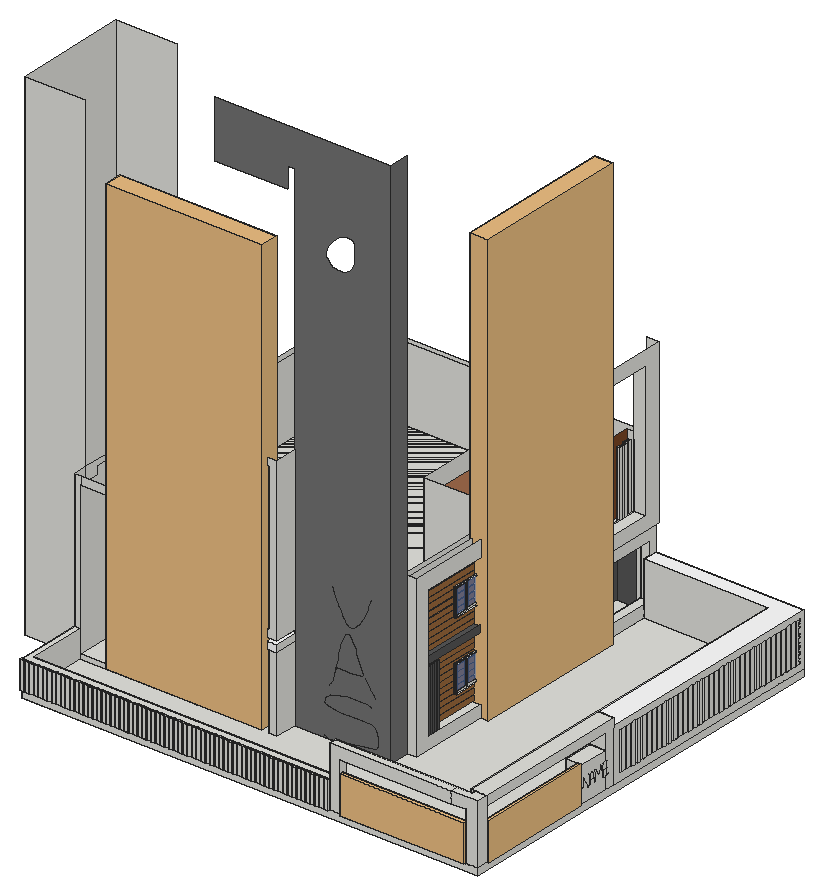
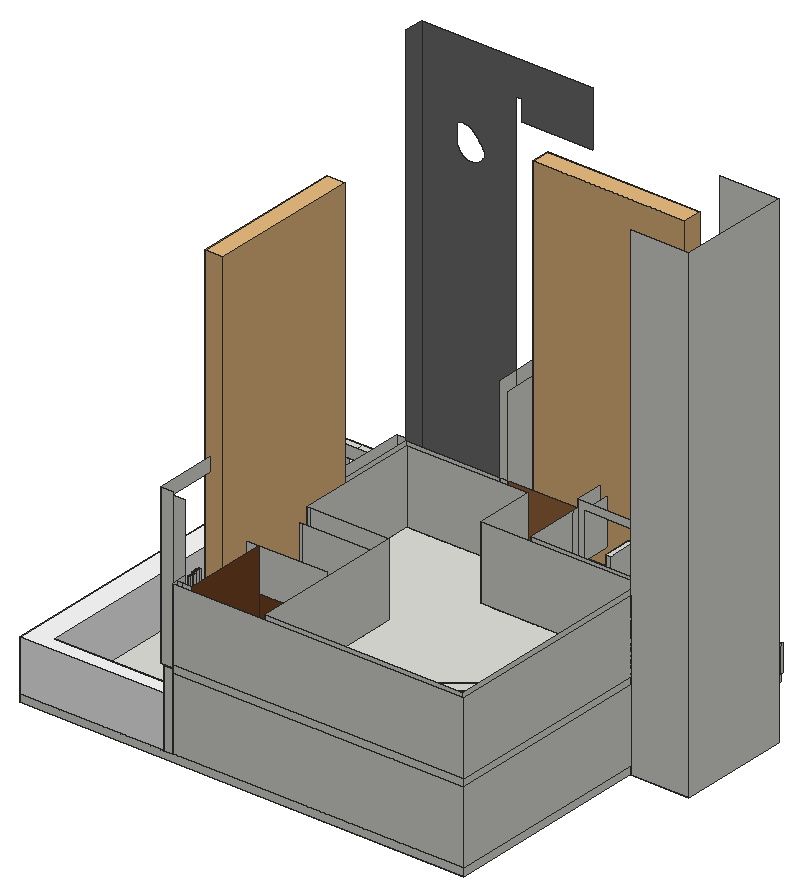
# SketchUp Ruby script. Lengths in inches.
U = 1.inch
M = Sketchup.active_model
def pt(a) = Geom::Point3d.new(a.map { |v| v * U })
def face(e, loops, mat)
  f = e.add_face(loops[0].map { |a| pt(a) })
  loops[1..].each { |l| e.add_face(l.map { |a| pt(a) }).erase! }
  f.material = f.back_material = mat if mat
  f
end
# faces: each face lists its corners as indices into pts; further lists are holes
def faces(e, pts, list, mat = nil) = list.each { |f| face(e, (f[0].is_a?(Array) ? f : [f]).map { |l| l.map { |i| pts[i] } }, mat) }
# xy, xz, yz: faces in a plane at the given z, y or x. An outline is a flat list of corners, or four numbers for a rectangle; further outlines are holes
def ring(l) = l.size == 4 ? [[l[0], l[1]], [l[2], l[1]], [l[2], l[3]], [l[0], l[3]]] : l.each_slice(2).to_a
def flat(e, list, mat, &to3) = list.each { |f| face(e, (f[0].is_a?(Array) ? f : [f]).map { |l| ring(l).map { |u, v| to3.(u, v) } }, mat) }
def xy(e, z, list, mat = nil) = flat(e, list, mat) { |x, y| [x, y, z] }
def xz(e, y, list, mat = nil) = flat(e, list, mat) { |x, z| [x, y, z] }
def yz(e, x, list, mat = nil) = flat(e, list, mat) { |y, z| [x, y, z] }
def lines(e, pts, list) = list.each { |a, b| e.add_line(pt(pts[a]), pt(pts[b])) }
# prism: a flat outline (further loops are holes) pulled along v
def prism(e, loops, v, mat = nil)
  f = face(e, loops, mat); d = Geom::Vector3d.new(v.map { |x| x * U })
  f.pushpull(f.normal.samedirection?(d) ? d.length : -d.length)
end
def box(e, o, s, mat = nil) = prism(e, [[o, [o[0] + s[0], o[1], o[2]], [o[0] + s[0], o[1] + s[1], o[2]], [o[0], o[1] + s[1], o[2]]]], [0, 0, s[2]], mat)
def at(x, y, z, deg = 0) = Geom::Transformation.translation(pt([x, y, z])) * Geom::Transformation.rotation(ORIGIN, Z_AXIS, deg.degrees)
def axes(o, x, y, z) = Geom::Transformation.new([*x, 0, *y, 0, *z, 0, *pt(o).to_a, 1])
def part(name) = M.definitions.add(name)
# library, detail: a bought-in or finely detailed component or shape, given as its bounding box
def library(name, o, s) = part(name).tap { |d| box(d.entities, o, s) }
def detail(e, o, s) = box(e.add_group.entities, o, s)
def put(e, d, t, mat = nil) = e.add_instance(d, t).tap { |i| i.material = mat if mat }
def group(e, t, mat = nil) = e.add_group.tap { |g| g.transformation = t; g.material = mat if mat }.entities
root = M.entities
M.materials.add("[Color M00]").color = [255, 255, 255]
M.materials.add("[Color M05]").color = [114, 114, 114]
M.materials.add("[Color M06]").color = [86, 86, 86]
M.materials.add("[Translucent Glass Blue]").color = [100, 149, 237]
M.materials["[Translucent Glass Blue]"].alpha = 0.5
M.materials.add("[Translucent_Glass_Gray]").color = [128, 128, 128]
M.materials["[Translucent_Glass_Gray]"].alpha = 0.5
M.materials.add("[Wood Floor]").color = [155, 105, 61]
M.materials.add("[Wood Veneer 01]").color = [120, 70, 37]
M.materials.add("[Wood Veneer 02]").color = [190, 128, 91]
c1 = library("House+plant_11",[-42.36,19.93,-20.98],[140.22,29.68,697.18])
c2 = part("Group\#13")
box(c2.entities,[0,-2.9375,0],[6.66,2.9375,44.375])
c3 = library("Group\#1076",[0,-1.74,0],[119.75,5.32,60.06])
c4 = part("Slatted corner screen")
put(c4.entities,c3,axes([-115.39,-96.71,0],[0,1.55247,0],[-1,0,0],[0,0,1]))
put(c4.entities,c3,axes([-334.41,-117.1,0],[1.66331,0,0],[0,1,0],[0,0,1]))
c5 = part("Group\#5")
xy(c5.entities,0,[[0,0,3.25,201.7]])
xy(c5.entities,8.11,[[0,0,3.25,201.7]])
xz(c5.entities,201.7,[[0,0,3.25,8.11]])
yz(c5.entities,3.25,[[0,0,201.7,8.11]])
c6 = part("Janela aluminio")
xy(c6.entities,0,[[0,0,47.24,1.57],[23.62,1.57,47.24,2.76],[0,2.76,25.98,3.9375],[0,3.9375,47.24,5.91]])
xy(c6.entities,43.31,[[0,0,47.24,1.57],[23.62,1.57,47.24,2.76],[0,2.76,0,5.91,47.24,5.91,47.24,3.9375,25.98,3.9375,25.98,2.76],[25.98,2.76,47.24,3.9375]])
xz(c6.entities,1.57,[[0,0,23.62,0,23.62,41.34,21.26,41.34,21.26,1.97,1.97,1.97,1.97,41.34,23.62,41.34,23.62,43.31,0,43.31],[[23.62,0,47.24,43.31],[25.7,1.97,45.28,41.34]]])
xz(c6.entities,2.76,[[[0,0,23.62,43.31],[2.36,2.36,21.26,40.94]],[23.62,0,25.98,43.31]])
xz(c6.entities,2.76,[[2.36,2.36,21.26,40.94]],"[Translucent Glass Blue]")
xz(c6.entities,3.9375,[[25.98,0,25.98,2.36,44.88,2.36,44.88,40.94,25.98,40.94,25.98,43.31,47.24,43.31,47.24,0]])
xz(c6.entities,3.9375,[[25.98,2.36,44.88,40.94]],"[Translucent Glass Blue]")
yz(c6.entities,0,[[0,0,1.57,43.31],[2.76,0,5.91,43.31]])
yz(c6.entities,23.62,[[1.57,0,2.76,43.31]])
yz(c6.entities,25.98,[[2.76,0,3.9375,43.31]])
yz(c6.entities,47.24,[[0,0,1.57,43.31],[1.57,0,2.76,43.31],[3.9375,0,5.91,43.31]])
c7 = part("Window frame")
prism(c7.entities,[[[0,70.87,0],[0,0,0],[0,0,47.24],[0,70.87,47.24]],[[0,1.97,1.97],[0,68.9,1.97],[0,68.9,45.28],[0,1.97,45.28]]],[7.875,0,0])
c8 = part("Window sash")
xy(c8.entities,0,[[0,0,3.9375,16.73]])
xy(c8.entities,0.98,[[0,0.98,1.77,15.75],[1.77,0.98,2.85,15.75],[2.85,0.98,3.9375,15.75]])
xy(c8.entities,42.32,[[0,0.98,1.77,15.75],[1.77,0.98,2.85,15.75],[2.85,0.98,3.9375,15.75]])
xy(c8.entities,43.31,[[0,0,3.9375,16.73]])
xz(c8.entities,0,[[0,0,3.9375,43.31]])
xz(c8.entities,0.98,[[0,0.98,1.77,42.32],[1.77,0.98,2.85,42.32],[2.85,0.98,3.9375,42.32]])
xz(c8.entities,15.75,[[0,0.98,1.77,42.32],[1.77,0.98,2.85,42.32],[2.85,0.98,3.9375,42.32]])
xz(c8.entities,16.73,[[0,0,3.9375,43.31]])
yz(c8.entities,0,[[[0,0,16.73,43.31],[0.98,0.98,15.75,42.32]]])
yz(c8.entities,1.77,[[0.98,0.98,15.75,42.32]],"[Translucent_Glass_Gray]")
yz(c8.entities,2.85,[[0.98,0.98,15.75,42.32]],"[Translucent_Glass_Gray]")
yz(c8.entities,3.9375,[[[0,0,16.73,43.31],[0.98,0.98,15.75,42.32]]])
c9 = part("simple window")
p = [[0,68.9,1.97],[0,35.43,1.97]]
lines(c9.entities,p,[[0,1]])
put(c9.entities,c7,at(0,0,0))
put(c9.entities,c8,axes([1.14,52.17,1.97],[0.71,0,0],[0,1,0],[0,0,1]))
put(c9.entities,c8,axes([1.14,1.97,1.97],[0.71,0,0],[0,1,0],[0,0,1]))
put(c9.entities,c8,axes([3.9375,18.7,1.97],[0.71,0,0],[0,1,0],[0,0,1]))
put(c9.entities,c8,axes([3.9375,35.43,1.97],[0.71,0,0],[0,1,0],[0,0,1]))
c10 = part("Group\#4")
box(c10.entities,[0,-480,0],[480,480,12])
c11 = part("Group\#12")
box(c11.entities,[0,0,-113.625],[4.125,3.0625,113.625])
xy(root,-12,[[0,129.5,96.8125,313.4]])
xy(root,-12,[[421.4,144.25,576.8125,176.625]],"[Color M05]")
xy(root,0,[[96.8125,2.9375,96.8125,108.5,105.7,108.5,105.7,15,590.66,15,590.66,2.9375],[590.66,2.9375,607.16,15.25],[810,2.9375,829.0625,21.875],[96.8125,108.5,286.44,176.625],[[409.15,108.5,421.4,108.5,421.4,176.625,591.75,176.625,591.75,656.625,576.8125,656.625,576.8125,400.39,441.125,400.39,441.125,509.52,537.25,509.52,537.25,647.625,576.8125,647.625,576.8125,656.625,96.8125,656.625,96.8125,185.625,105.8125,185.625,105.8125,273.5625,293.58,273.5625,293.58,176.625,409.15,176.625],[368.4,185.625,368.4,282.5625,105.8125,282.5625,105.8125,647.625,432.125,647.625,432.125,391.39,567.8125,391.39,567.8125,185.625]],
  [96.8125,176.625,105.8125,185.625],[368.4,185.625,567.8125,185.625,567.8125,391.39,432.125,391.39,432.125,647.625,105.8125,647.625,105.8125,282.5625,368.4,282.5625],[802.8125,212.39,829.0625,260.08],[802.8125,260.08,829.0625,276.46],[441.125,400.39,567.8125,400.39,567.8125,647.625,537.25,647.625,537.25,509.52,551.125,509.52,551.125,496.2,441.125,496.2],
  [567.8125,400.39,576.8125,647.625],[591.75,632.64,790.44,656.625]])
xy(root,0,[[286.44,108.5,293.58,141.5625]],"[Color M00]")
xy(root,7.8125,[[107.25,108.5,293.58,108.5,293.58,185.625,96.8125,185.625,96.8125,176.75,107.25,176.75]])
xy(root,10.33,[[819.0625,286.78,819.0625,646.3,829.0625,646.3,829.0625,297.7,821.875,297.7,821.875,292.02,829.0625,292.02,829.0625,286.78],[821.875,292.02,829.0625,297.7]])
xy(root,18.83,[[576.8125,198.69,591.75,644.4375]])
xy(root,43,[[286.44,108.5,293.58,176.625]],"[Color M00]")
xy(root,44.375,[[96.8125,2.9375,590.66,2.9375,590.66,15,105.7,15,105.7,108.5,96.8125,108.5]])
xy(root,53.625,[[441.125,496.2,551.125,509.52]])
xy(root,56,[[802.8125,212.39,829.0625,260.08]])
xy(root,60.625,[[576.8125,386.37,591.75,400.39]])
xy(root,62.1875,[[238.96,108.5,248.39,176.625]],"[Color M00]")
xy(root,74.24,[[819.0625,286.78,829.0625,286.78,829.0625,292.02,821.875,292.02,821.875,297.7,829.0625,297.7,829.0625,646.3,819.0625,646.3],[821.875,292.02,829.0625,297.7]])
xy(root,77.84,[[607.16,2.9375,810,15.25]])
xy(root,81.34,[[802.8125,21.875,829.0625,260.08]])
xy(root,84.5625,[[790.44,276.46,790.44,632.64,591.75,632.64,591.75,656.625,829.0625,656.625,829.0625,276.46]],"[Color M00]")
xy(root,96.09,[[590.66,2.9375,786.3125,15.25],[786.3125,2.9375,829.0625,2.9375,829.0625,21.875,810,21.875,810,15.25,786.3125,15.25],[802.8125,21.875,829.0625,276.46]])
xy(root,105.25,[[576.8125,400.39,591.75,644.4375]])
xy(root,120,[[[409.15,108.5,421.4,108.5,421.4,176.625,576.8125,176.625,576.8125,400.39,441.125,400.39,441.125,509.52,537.25,509.52,537.25,647.625,576.8125,647.625,576.8125,656.625,96.8125,656.625,96.8125,176.75,105.8125,176.75,105.8125,273.5625,293.58,273.5625,293.58,176.625,409.15,176.625],[368.4,185.625,368.4,282.5625,105.8125,282.5625,105.8125,647.625,432.125,647.625,432.125,391.39,567.8125,391.39,567.8125,185.625]],[96.8125,176.625,105.8125,176.75]])
xy(root,120,[[248.39,108.5,409.15,176.625]],"[Color M00]")
xy(root,120,[[576.8125,198.69,589.375,386.37]],"[Color M06]")
xy(root,125.71,[[576.8125,386.37,591.75,656.625]])
xy(root,127.5625,[[576.8125,386.37,596.375,656.625]])
xy(root,132,[[[96.8125,176.625,105.8125,176.625,105.8125,273.5625,293.58,273.5625,293.58,176.625,576.8125,176.625,576.8125,400.39,441.125,400.39,441.125,509.52,552.625,509.52,552.625,647.625,576.8125,647.625,576.8125,656.625,96.8125,656.625],[368.4,185.625,368.4,282.5625,105.8125,282.5625,105.8125,647.625,432.125,647.625,432.125,391.39,567.8125,391.39,567.8125,185.625]],[105.8125,176.625,293.58,273.5625],[368.4,185.625,567.8125,185.625,567.8125,391.39,432.125,391.39,432.125,647.625,105.8125,647.625,105.8125,282.5625,368.4,282.5625],[441.125,400.39,567.8125,400.39,567.8125,647.625,552.625,647.625,552.625,509.52,441.125,509.52],[567.8125,400.39,576.8125,647.625]])
xy(root,132,[[238.96,108.5,421.4,176.625]],"[Color M00]")
xy(root,132,[[576.8125,198.69,589.375,386.37]],"[Color M06]")
xy(root,136.75,[[238.96,108.5,421.4,176.625]])
xy(root,148.6875,[[576.8125,400.39,596.375,631.75]])
xy(root,149.72,[[247.29,108.5,408.47,176.625]])
xy(root,175.98,[[294.92,105.68,282.85,105.86,283.87,173.99,295.94,173.81]])
xy(root,181.38,[[441.125,495.37,591.75,509.52]])
xy(root,192.45,[[576.8125,386.37,596.375,400.39]])
xy(root,200.03,[[238.96,108.5,247.29,176.625]])
xz(root,2.9375,[[96.8125,0,584,44.375],[590.66,0,607.16,0,607.16,77.84,786.3125,77.84,786.3125,96.09,590.66,96.09],[810,0,829.0625,0,829.0625,96.09,786.3125,96.09,786.3125,77.84,810,77.84]])
xz(root,15,[[105.7,0,590.66,44.375]])
xz(root,15.25,[[590.66,0,590.66,96.09,810,96.09,810,77.84,607.16,77.84,607.16,0]])
xz(root,21.875,[[810,0,829.0625,81.34],[802.8125,81.34,810,96.09],[810,81.34,829.0625,96.09]])
xz(root,108.5,[[105.7,0,286.44,0,286.44,7.8125,107.25,7.8125,107.25,264,96.8125,264,96.8125,44.375,105.7,44.375],[409.15,0,421.4,120],[238.96,136.75,421.4,136.75,421.4,396,238.96,396,238.96,328.5625,250.4375,328.5625,250.4375,384,408.47,384,408.47,149.72,247.29,149.72,247.29,200.03,238.96,200.03]])
xz(root,108.5,[[286.44,0,293.58,7.8125],[286.44,7.8125,293.58,43],[238.96,62.1875,238.96,132,421.4,132,421.4,120,248.39,120,248.39,62.1875]],"[Color M00]")
xz(root,129.5,[[0,-12,96.8125,792]])
xz(root,144.25,[[[421.4,-12,576.8125,-12,576.8125,859.0625,293.58,859.0625,293.58,767.74,411.47,767.74,411.47,801.24,421.4,801.24],[499.28,678.61,496.52,678.68,493.5,678.8,491.18,678.99,488.85,679.28,486.04,679.74,483.9,680.62,481.86,681.66,480.42,683.44,478.12,684.95,476.52,686.92,475.09,689.5,473.78,691.2,472.16,693.875,472.29,696.5,472.54,698.74,472.87,700.99,473.375,703.48,474.84,705.29,475.72,707.47,477,709.55,478.57,711.1,479.9,713.53,481.51,715.31,482.91,717.36,484.83,719.08,486.18,720.94,488.32,722.59,489.21,724.33,494.25,727.71,498.73,730.52,506.22,732.9,508.87,732.625,511.41,732.18,513.8,731.55,515.96,730.33,517.58,728.38,518.67,726.53,519.03,723.43,519.05,720.89,519.07,717.8,519.08,715.27,519.08,712.16,519.06,709.68,519.01,706.6,518.93,703.9,518.75,701.49,518.48,698.83,518.06,696.2,517.19,693.71,515.95,691.83,514.6,689.38,512.91,687.64,511.65,685.61,509.4,683.71,507.3125,682.48,504.6,680.79,502.39,679.59],[488.29,106.62,488.6,110.46,490.04,114.3,490.41,118.74,490.65,123.21,490.87,127.17,492.64,132.22,494.14,136.88,494.63,140.95,496.73,145.54,497.9,149.01,500.61,154.49,502.59,158.07,505.04,161.36,508.8,162.92,512.82,158.32,515.375,155.08,517.24,151.33,519.4,146.99,520.85,142.62,522.12,138.13,523.31,134.68,525.51,130.3,526.77,126.94,527.37,123.24,530.09,118.92,531.4,115.1,532.57,110.72,535.46,107.9,512.74,106.76,501.53,106.76],[551.45,10.1875,552.47,11.31,557.07,12]],[551.45,10.1875,557.07,12,552.47,11.31],[488.29,106.62,501.53,106.76,512.74,106.76,535.46,107.9,532.57,110.72,531.4,115.1,530.09,118.92,527.37,123.24,526.77,126.94,525.51,130.3,523.31,134.68,522.12,138.13,520.85,142.62,519.4,146.99,517.24,151.33,515.375,155.08,512.82,158.32,508.8,162.92,505.04,161.36,502.59,158.07,500.61,154.49,497.9,149.01,496.73,145.54,494.63,140.95,494.14,136.88,492.64,132.22,490.87,127.17,490.65,123.21,490.41,118.74,490.04,114.3,488.6,110.46]],"[Color M05]")
xz(root,176.625,[[421.4,-12,576.8125,0],[96.8125,0,105.8125,120],[421.4,0,576.8125,120],[576.8125,0,591.75,256.375],[96.8125,120,105.8125,132],
  [421.4,120,576.8125,132],[96.8125,132,105.8125,252],[421.4,132,576.8125,252],[238.96,136.75,238.96,200.03,247.29,200.03,247.29,149.72,293.58,149.72,293.58,136.75],[293.58,136.75,421.4,136.75,421.4,252,408.47,252,408.47,149.72,293.58,149.72]])
xz(root,176.625,[[238.96,62.1875,248.39,120]],"[Color M00]")
xz(root,176.625,[[293.58,0,409.15,120],[293.58,132,421.4,136.75],[293.58,149.72,408.47,252]],"[Wood Floor]")
xz(root,176.75,[[96.8125,7.8125,96.8125,120,105.8125,120,105.8125,264,107.25,264,107.25,7.8125]])
xz(root,185.625,[[96.8125,0,105.8125,7.8125],[105.8125,0,293.58,7.8125],[368.4,0,567.8125,120],[368.4,132,567.8125,252]])
xz(root,198.69,[[576.8125,18.83,576.8125,120,589.375,120,589.375,132,576.8125,132,576.8125,218.23,580.0625,218.23,580.0625,226.34,576.8125,226.34,576.8125,230.57,591.75,230.57,591.75,18.83],[576.8125,120,589.375,132],[576.8125,218.23,580.0625,226.34]])
xz(root,212.39,[[802.8125,0,829.0625,56]])
xz(root,260.08,[[802.8125,0,829.0625,56],[802.8125,56,829.0625,81.34]])
xz(root,273.5625,[[105.8125,0,293.58,120],[105.8125,132,293.58,252]])
xz(root,276.46,[[790.44,0,802.8125,84.5625],[802.8125,0,829.0625,84.5625],[802.8125,84.5625,829.0625,96.09]])
xz(root,282.5625,[[105.8125,0,368.4,120],[105.8125,132,368.4,252]])
xz(root,286.78,[[819.0625,10.33,829.0625,74.24]])
xz(root,292.02,[[821.875,10.33,829.0625,74.24]])
xz(root,297.7,[[821.875,10.33,829.0625,74.24]])
xz(root,302.39,[[821.875,10.33,829.0625,74.24]])
xz(root,308.08,[[821.875,10.33,829.0625,74.24]])
xz(root,312.77,[[821.875,10.33,829.0625,74.24]])
xz(root,313.4,[[0,-12,96.8125,792]])
xz(root,318.45,[[821.875,10.33,829.0625,74.24]])
xz(root,323.14,[[821.875,10.33,829.0625,74.24]])
xz(root,328.83,[[821.875,10.33,829.0625,74.24]])
xz(root,333.52,[[821.875,10.33,829.0625,74.24]])
xz(root,339.2,[[821.875,10.33,829.0625,74.24]])
xz(root,343.89,[[821.875,10.33,829.0625,74.24]])
xz(root,349.58,[[821.875,10.33,829.0625,74.24]])
xz(root,354.27,[[821.875,10.33,829.0625,74.24]])
xz(root,359.95,[[821.875,10.33,829.0625,74.24]])
xz(root,364.64,[[821.875,10.33,829.0625,74.24]])
xz(root,370.33,[[821.875,10.33,829.0625,74.24]])
xz(root,375.02,[[821.875,10.33,829.0625,74.24]])
xz(root,380.7,[[821.875,10.33,829.0625,74.24]])
xz(root,385.39,[[821.875,10.33,829.0625,74.24]])
xz(root,386.37,[[576.8125,60.625,591.75,60.625,591.75,125.71,589.375,125.71,589.375,120,576.8125,120],[576.8125,120,589.375,125.71],[576.8125,125.71,589.375,127.5625],[576.8125,127.5625,589.375,132],[589.375,127.5625,596.375,127.5625,596.375,192.45,576.8125,192.45,576.8125,132,589.375,132]])
xz(root,391.08,[[821.875,10.33,829.0625,74.24]])
xz(root,391.39,[[432.125,0,562.8125,120],[562.8125,0,567.8125,120],[432.125,132,562.8125,252],[562.8125,132,567.8125,252]])
xz(root,395.77,[[821.875,10.33,829.0625,74.24]])
xz(root,400.39,[[441.125,0,567.8125,120],[567.8125,0,576.8125,120],[576.8125,60.625,591.75,105.25],[441.125,132,567.8125,230.57],[567.8125,132,576.8125,230.57],
  [576.8125,148.6875,596.375,192.45]])
xz(root,401.45,[[821.875,10.33,829.0625,74.24]])
xz(root,406.14,[[821.875,10.33,829.0625,74.24]])
xz(root,411.83,[[821.875,10.33,829.0625,74.24]])
xz(root,416.52,[[821.875,10.33,829.0625,74.24]])
xz(root,422.2,[[821.875,10.33,829.0625,74.24]])
xz(root,426.89,[[821.875,10.33,829.0625,74.24]])
xz(root,432.58,[[821.875,10.33,829.0625,74.24]])
xz(root,437.27,[[821.875,10.33,829.0625,74.24]])
xz(root,442.95,[[821.875,10.33,829.0625,74.24]])
xz(root,447.64,[[821.875,10.33,829.0625,74.24]])
xz(root,453.33,[[821.875,10.33,829.0625,74.24]])
xz(root,458.02,[[821.875,10.33,829.0625,74.24]])
xz(root,463.7,[[821.875,10.33,829.0625,74.24]])
xz(root,468.39,[[821.875,10.33,829.0625,74.24]])
xz(root,474.08,[[821.875,10.33,829.0625,74.24]])
xz(root,478.77,[[821.875,10.33,829.0625,74.24]])
xz(root,484.45,[[821.875,10.33,829.0625,74.24]])
xz(root,489.14,[[821.875,10.33,829.0625,74.24]])
xz(root,494.83,[[821.875,10.33,829.0625,74.24]])
xz(root,495.37,[[441.125,181.38,591.75,230.57]])
xz(root,496.2,[[441.125,0,551.125,53.625]])
xz(root,499.52,[[821.875,10.33,829.0625,74.24]])
xz(root,505.2,[[821.875,10.33,829.0625,74.24]])
xz(root,509.52,[[441.125,0,537.25,53.625],[537.25,0,551.125,53.625],[441.125,181.38,552.625,252],[552.625,181.38,552.625,252,576.8125,252,576.8125,256.375,591.75,256.375,591.75,181.38]])
xz(root,509.52,[[441.125,53.625,537.25,120]],"[Color M06]")
xz(root,509.52,[[441.125,132,552.625,181.38]],"[Wood Veneer 01]")
xz(root,509.95,[[821.875,10.33,829.0625,74.24]])
xz(root,515.64,[[821.875,10.33,829.0625,74.24]])
xz(root,520.39,[[821.875,10.33,829.0625,74.24]])
xz(root,526.08,[[821.875,10.33,829.0625,74.24]])
xz(root,530.83,[[821.875,10.33,829.0625,74.24]])
xz(root,536.52,[[821.875,10.33,829.0625,74.24]])
xz(root,541.27,[[821.875,10.33,829.0625,74.24]])
xz(root,546.95,[[821.875,10.33,829.0625,74.24]])
xz(root,551.7,[[821.875,10.33,829.0625,74.24]])
xz(root,557.39,[[821.875,10.33,829.0625,74.24]])
xz(root,562.14,[[821.875,10.33,829.0625,74.24]])
xz(root,567.83,[[821.875,10.33,829.0625,74.24]])
xz(root,572.58,[[821.875,10.33,829.0625,74.24]])
xz(root,578.27,[[821.875,10.33,829.0625,74.24]])
xz(root,583.02,[[821.875,10.33,829.0625,74.24]])
xz(root,588.7,[[821.875,10.33,829.0625,74.24]])
xz(root,593.45,[[821.875,10.33,829.0625,74.24]])
xz(root,599.14,[[821.875,10.33,829.0625,74.24]])
xz(root,603.89,[[821.875,10.33,829.0625,74.24]])
xz(root,609.58,[[821.875,10.33,829.0625,74.24]])
xz(root,613.7,[[821.875,10.33,829.0625,74.24]])
xz(root,619.39,[[821.875,10.33,829.0625,74.24]])
xz(root,623.52,[[821.875,10.33,829.0625,74.24]])
xz(root,629.2,[[821.875,10.33,829.0625,74.24]])
xz(root,631.75,[[576.8125,148.6875,596.375,365.16]])
xz(root,632.64,[[591.75,0,790.44,84.5625]])
xz(root,633.33,[[821.875,10.33,829.0625,74.24]])
xz(root,639.02,[[821.875,10.33,829.0625,74.24]])
xz(root,643.14,[[821.875,10.33,829.0625,74.24]])
xz(root,644.4375,[[576.8125,18.83,591.75,105.25]])
xz(root,646.3,[[819.0625,10.33,829.0625,74.24]])
xz(root,647.625,[[105.8125,0,432.125,120],[567.8125,0,576.8125,120],[105.8125,132,432.125,252],[552.625,132,567.8125,252],[567.8125,132,576.8125,252]])
xz(root,647.625,[[537.25,0,567.8125,120]],"[Color M06]")
xz(root,648.83,[[821.875,10.33,829.0625,74.24]])
xz(root,656.625,[[96.8125,0,576.8125,120],[576.8125,0,591.75,125.71],[576.8125,127.5625,596.375,387.92],[96.8125,132,576.8125,252]])
xz(root,656.625,[[591.75,0,829.0625,84.5625]],"[Color M00]")
yz(root,0,[[129.5,-12,313.4,792]])
yz(root,96.8125,[[129.5,-12,313.4,0],[2.9375,0,108.5,44.375],[108.5,0,129.5,264],[129.5,0,176.625,7.8125],[176.625,0,185.625,7.8125],
  [313.4,0,656.625,120],[129.5,7.8125,176.625,24.43],[176.625,7.8125,176.75,24.43],[129.5,24.43,176.625,264],[176.625,24.43,176.75,120],
  [176.625,120,176.75,132],[176.75,120,313.4,132],[176.625,132,176.75,252],[176.75,132,313.4,252],[313.4,132,656.625,252]])
yz(root,105.7,[[15,0,108.5,44.375]])
yz(root,105.8125,[[176.625,0,273.5625,120],[282.5625,0,647.625,120],[176.625,120,176.75,132],[176.625,132,176.75,252],[176.75,132,273.5625,252],
  [282.5625,132,647.625,252]])
yz(root,107.25,[[108.5,7.8125,176.75,7.8125,176.75,264,141.5625,264,141.5625,251.42,108.5,251.42]])
yz(root,238.96,[[108.5,136.75,176.625,200.03]])
yz(root,238.96,[[108.5,62.1875,176.625,132]],"[Color M00]")
yz(root,247.29,[[108.5,149.72,176.625,200.03]])
yz(root,248.39,[[108.5,62.1875,176.625,120]],"[Color M00]")
yz(root,286.44,[[108.5,0,176.625,43]],"[Color M00]")
yz(root,293.58,[[108.5,0,176.625,7.8125],[176.625,0,185.625,7.8125],[185.625,0,273.5625,120],[176.625,7.8125,185.625,120],[176.625,132,185.625,252],
  [185.625,132,273.5625,252]])
yz(root,293.58,[[108.5,7.8125,176.625,43]],"[Color M00]")
yz(root,368.4,[[185.625,0,282.5625,120],[185.625,132,282.5625,252]])
yz(root,408.47,[[108.5,149.72,176.625,384]])
yz(root,409.15,[[108.5,0,176.625,120]])
yz(root,421.4,[[108.5,0,144.25,120],[108.5,120,144.25,132],[108.5,136.75,144.25,396],[144.25,136.75,176.625,396]])
yz(root,421.4,[[144.25,-12,176.625,0],[144.25,0,176.625,120],[144.25,120,176.625,132],[144.25,132,176.625,136.75]],"[Color M05]")
yz(root,432.125,[[391.39,0,647.625,120],[391.39,132,647.625,252]])
yz(root,441.125,[[496.2,0,509.52,53.625]])
yz(root,441.125,[[400.39,0,496.2,0,496.2,53.625,509.52,53.625,509.52,120,400.39,120],[400.39,132,509.52,132,509.52,181.38,495.37,181.38,495.37,230.57,400.39,230.57]],"[Wood Veneer 02]")
yz(root,537.25,[[509.52,0,647.625,120]],"[Color M06]")
yz(root,551.125,[[496.2,0,509.52,53.625]])
yz(root,552.625,[[509.52,132,647.625,252]],"[Wood Veneer 01]")
yz(root,567.8125,[[185.625,0,391.39,120],[185.625,132,391.39,252]])
yz(root,576.8125,[[400.39,0,647.625,18.83],[647.625,0,656.625,120],[198.69,18.83,400.39,18.83,400.39,60.625,386.37,60.625,386.37,120,198.69,120],[644.4375,18.83,647.625,114.5625],[386.37,60.625,400.39,120],
  [400.39,105.25,644.4375,105.25,644.4375,114.5625,647.625,114.5625,647.625,120,656.625,120,656.625,125.71,386.37,125.71,386.37,120,400.39,120],[176.625,120,198.69,132],[386.37,127.5625,656.625,132],[176.625,132,198.69,132,198.69,230.57,400.39,230.57,400.39,252,176.625,252],[198.69,132,386.37,132,386.37,192.45,400.39,192.45,400.39,218.23,198.69,218.23],
  [400.39,132,631.75,148.6875],[631.75,132,647.625,134.98],[647.625,132,656.625,252],[631.75,134.98,647.625,252],[198.69,218.23,400.39,226.34]])
yz(root,576.8125,[[144.25,-12,176.625,859.0625]],"[Color M05]")
yz(root,589.375,[[198.69,120,386.37,132]],"[Color M06]")
yz(root,590.66,[[2.9375,0,15,44.375],[15,0,15.25,44.375],[2.9375,44.375,15.25,96.09]])
yz(root,591.75,[[176.625,0,632.64,0,632.64,18.83,198.69,18.83,198.69,230.57,495.37,230.57,495.37,181.38,509.52,181.38,509.52,256.375,176.625,256.375],[632.64,0,656.625,0,656.625,84.5625,644.4375,84.5625,644.4375,18.83,632.64,18.83],[632.64,18.83,644.4375,84.5625],[386.37,60.625,400.39,60.625,400.39,105.25,644.4375,105.25,644.4375,84.5625,656.625,84.5625,656.625,125.71,386.37,125.71]])
yz(root,596.375,[[386.37,127.5625,656.625,127.5625,656.625,387.92,385.5625,387.92,385.5625,331.1,400.39,331.1,400.39,365.16,631.75,365.16,631.75,148.6875,400.39,148.6875,400.39,192.45,386.37,192.45]])
yz(root,607.16,[[2.9375,0,15.25,77.84]])
yz(root,790.44,[[276.46,0,632.64,84.5625]],"[Color M00]")
yz(root,802.8125,[[260.08,0,260.08,81.34,21.875,81.34,21.875,96.09,276.46,96.09,276.46,0],[212.39,0,260.08,56]])
yz(root,810,[[2.9375,0,2.9375,77.84,15.25,77.84,15.25,96.09,21.875,96.09,21.875,0]])
yz(root,819.0625,[[286.78,10.33,646.3,74.24]])
yz(root,821.875,[[292.02,10.33,297.7,74.24]])
yz(root,829.0625,[[2.9375,0,21.875,96.09],[260.08,0,276.46,0,276.46,96.09,21.875,96.09,21.875,81.34,260.08,81.34],[212.39,0,260.08,0,260.08,20.7,259.9375,20.67,258.65,20.28,257.54,19.92,256.68,19.77,256.32,19.96,256.24,20.25,256.19,20.82,256.14,21.54,256.05,22.53,255.79,23.68,255.63,24.96,255.4375,26.42,255.04,28.42,254.7,30.78,254.47,32.5,254.1,35.04,253.7,37.43,253.68,38.35,253.5,39.45,253.51,40.39,253.78,40.36,254.89,40.46,255.24,40.67,255.58,40.71,256.01,40.76,256.61,40.85,257.76,41.04,259.65,41.16,260.08,41.21,260.08,56,212.39,56],[[276.46,0,656.625,84.5625],[286.78,10.33,646.3,74.24]],[292.02,10.33,297.7,74.24],
  [302.39,10.33,308.08,74.24],[312.77,10.33,318.45,74.24],[323.14,10.33,328.83,74.24],[333.52,10.33,339.2,74.24],[343.89,10.33,349.58,74.24],
  [354.27,10.33,359.95,74.24],[364.64,10.33,370.33,74.24],[375.02,10.33,380.7,74.24],[385.39,10.33,391.08,74.24],[395.77,10.33,401.45,74.24],
  [406.14,10.33,411.83,74.24],[416.52,10.33,422.2,74.24],[426.89,10.33,432.58,74.24],[437.27,10.33,442.95,74.24],[447.64,10.33,453.33,74.24],
  [458.02,10.33,463.7,74.24],[468.39,10.33,474.08,74.24],[478.77,10.33,484.45,74.24],[489.14,10.33,494.83,74.24],[499.52,10.33,505.2,74.24],
  [509.95,10.33,515.64,74.24],[520.39,10.33,526.08,74.24],[530.83,10.33,536.52,74.24],[541.27,10.33,546.95,74.24],[551.7,10.33,557.39,74.24],
  [562.14,10.33,567.83,74.24],[572.58,10.33,578.27,74.24],[583.02,10.33,588.7,74.24],[593.45,10.33,599.14,74.24],[603.89,10.33,609.58,74.24],
  [613.7,10.33,619.39,74.24],[623.52,10.33,629.2,74.24],[633.33,10.33,639.02,74.24],[643.14,10.33,646.3,74.24],[646.3,10.33,648.83,74.24],
  [256.68,19.77,257.54,19.92,258.65,20.28,259.9375,20.67,260.08,20.7,260.08,41.21,259.65,41.16,257.76,41.04,256.61,40.85,256.01,40.76,255.58,40.71,255.24,40.67,254.89,40.46,253.78,40.36,253.51,40.39,253.5,39.45,253.68,38.35,253.7,37.43,254.1,35.04,254.47,32.5,254.7,30.78,255.04,28.42,255.4375,26.42,255.63,24.96,255.79,23.68,256.05,22.53,256.14,21.54,256.19,20.82,256.24,20.25,256.32,19.96]])
p = [[106.75,108.5,264],[106.75,108.5,251.42],[106.76,108.5,251.42],[282.85,105.86,251.42],[282.85,105.86,175.98],[294.92,105.68,175.98],
  [294.92,105.68,264],[106.76,108.5,264],[295.94,173.81,264],[295.94,173.81,175.98],[283.87,173.99,251.42],[283.87,173.99,175.98],
  [107.78,176.625,251.42],[107.78,176.625,264],[482.51,144.25,222.04],[483.57,144.25,218.43],[485.2,144.25,213.03],[487.05,144.25,208.95],
  [488.81,144.25,205.01],[491.2,144.25,199.92],[493.17,144.25,195.31],[495.66,144.25,192.37],[497.72,144.25,188.57],[499.15,144.25,184.26],
  [502.13,144.25,180.49],[503.65,144.25,176.69],[506.64,144.25,174],[510.48,144.25,172.15],[515.05,144.25,172.25],[518.87,144.25,174.61],
  [523.24,144.25,179.375],[526.62,144.25,182.25],[528.67,144.25,185.21],[530.95,144.25,189.92],[533.61,144.25,193.12],[535.67,144.25,198.43],
  [537.68,144.25,202.52],[539.66,144.25,206.97],[540.4375,144.25,211.59],[541.54,144.25,216.15],[543.69,144.25,220.2],[544.86,144.25,223.6],
  [477.35,144.25,77.7],[482.93,144.25,85.21],[485.7,144.25,95.53],[485.6875,144.25,98.34],[487.63,144.25,101.8],[488.29,144.25,106.62],
  [535.46,144.25,107.9],[536.86,144.25,104.27],[539.23,144.25,101.13],[542.4,144.25,96.48],[544.55,144.25,92.62],[547.23,144.25,89.9375],
  [549.43,144.25,86.86],[552.05,144.25,83.9],[545.69,144.25,68.24],[537.25,144.25,71.07],[526.96,144.25,71.08],[524.25,144.25,70.8],
  [520.71,144.25,71.03],[515.89,144.25,71.05],[511.5,144.25,71.05],[506.98,144.25,71.08],[501.79,144.25,69.96],[497.62,144.25,68.61],
  [493.01,144.25,68.24],[488.35,144.25,66.23],[483.18,144.25,64.53],[478.41,144.25,63.95],[475.92,144.25,61.21],[472.18,144.25,59.31],
  [470.72,144.25,54.64],[469.82,144.25,50.42],[474.74,144.25,47.78],[480.54,144.25,46.36],[485.47,144.25,45.39],[490.34,144.25,44.78],
  [494.08,144.25,44.42],[498.61,144.25,44.1875],[503.19,144.25,44.04],[508.86,144.25,44.51],[513.72,144.25,44.57],[517.96,144.25,44.61],
  [522.68,144.25,44.67],[527.9,144.25,44.68],[531.53,144.25,44.7],[536.62,144.25,44.7],[541.34,144.25,44.7],[545.4,144.25,44.7],
  [550.02,144.25,41.875],[552.4,144.25,39.04],[554.33,144.25,35.37],[555.44,144.25,30.67],[556.11,144.25,26.8125],[556.5625,144.25,22.37],
  [556.29,144.25,17.23],[554.11,144.25,13.1],[552.47,144.25,11.31],[477.61,144.25,0],[469.18,144.25,3.28],[829.0625,213.49,22.12],
  [829.0625,213.49,23.01],[829.0625,213.84,24.08],[829.0625,213.82,24.37],[829.0625,213.85,25.05],[829.0625,213.89,25.64],[829.0625,213.89,26.07],
  [829.0625,213.9,26.56],[829.0625,213.91,27.08],[829.0625,213.91,27.43],[829.0625,213.91,27.93],[829.0625,213.91,28.65],[829.0625,213.91,29.42],
  [829.0625,213.91,30.23],[829.0625,213.9,30.86],[829.0625,213.9,31.63],[829.0625,213.9,32.3],[829.0625,213.9,33.01],[829.0625,213.9,33.5625],
  [829.0625,214,34.1875],[829.0625,214.08,34.65],[829.0625,214.15,35.03],[829.0625,214.1875,35.53],[829.0625,214.21,35.93],[829.0625,214.38,36.37],
  [829.0625,214.58,36.66],[829.0625,215.07,36.58],[829.0625,215.42,36.26],[829.0625,215.83,35.68],[829.0625,216.37,34.24],[829.0625,216.77,33.53],
  [829.0625,217.27,32.17],[829.0625,218.05,30.82],[829.0625,218.94,29.54],[829.0625,219.89,28.04],[829.0625,220.57,26.88],[829.0625,221.06,26.32],
  [829.0625,221.58,25.24],[829.0625,221.91,24.42],[829.0625,222.19,23.72],[829.0625,222.4375,23.01],[829.0625,222.55,22.5],[829.0625,222.625,22.15],
  [829.0625,222.68,21.74],[829.0625,222.7,21.36],[829.0625,222.78,20.99],[829.0625,222.96,20.57],[829.0625,223.12,20.25],[829.0625,223.33,19.94],
  [829.0625,223.73,19.81],[829.0625,224.12,19.72],[829.0625,224.47,19.87],[829.0625,225,20.14],[829.0625,225.45,20.74],[829.0625,225.84,21.38],
  [829.0625,226.01,21.98],[829.0625,226.13,22.38],[829.0625,226.21,22.97],[829.0625,226.26,23.72],[829.0625,226.29,24.51],[829.0625,226.3,25.39],
  [829.0625,226.3125,26.27],[829.0625,226.32,27.25],[829.0625,226.32,27.79],[829.0625,226.33,28.84],[829.0625,226.33,29.96],[829.0625,226.33,30.88],
  [829.0625,226.32,32.09],[829.0625,226.32,33.35],[829.0625,226.22,34.19],[829.0625,226.03,35.09],[829.0625,225.875,35.75],[829.0625,225.71,36.28],
  [829.0625,225.58,36.75],[829.0625,225.53,37.08],[829.0625,225.49,37.46],[829.0625,225.46,37.83],[829.0625,228.4,21.24],[829.0625,228.4,22.14],
  [829.0625,228.4,23.22],[829.0625,228.51,23.5625],[829.0625,228.53,24.96],[829.0625,228.55,25.65],[829.0625,228.5625,26.72],[829.0625,228.57,27.68],
  [829.0625,228.57,28.59],[829.0625,228.57,29.52],[829.0625,228.58,30.22],[829.0625,228.58,30.92],[829.0625,228.58,31.38],[829.0625,228.58,32.1],
  [829.0625,228.74,32.6875],[829.0625,228.82,33.46],[829.0625,228.91,34.08],[829.0625,229.01,34.77],[829.0625,229.26,35.37],[829.0625,229.33,35.95],
  [829.0625,229.43,36.41],[829.0625,229.7,36.89],[829.0625,229.77,37.36],[829.0625,229.99,37.82],[829.0625,230.17,38.12],[829.0625,230.51,38.38],
  [829.0625,230.89,38.51],[829.0625,231.23,38.64],[829.0625,231.59,38.71],[829.0625,232,38.7],[829.0625,232.32,38.34],[829.0625,232.95,37.46],
  [829.0625,233.48,36.65],[829.0625,233.89,35.76],[829.0625,234.26,34.6],[829.0625,234.75,33.22],[829.0625,234.98,32.58],[829.0625,235.27,31.44],
  [829.0625,235.41,30.74],[829.0625,235.59,29.39],[829.0625,235.94,27.9],[829.0625,236.32,26.53],[829.0625,236.61,25.33],[829.0625,236.85,24.31],
  [829.0625,236.96,23.42],[829.0625,237.04,22.96],[829.0625,237.25,22.19],[829.0625,237.32,21.79],[829.0625,237.41,21.375],[829.0625,237.46,20.96],
  [829.0625,237.48,20.52],[829.0625,229.48,27.72],[829.0625,230.92,27.71],[829.0625,232.28,27.71],[829.0625,232.35,27.71],[829.0625,232.7,27.71],
  [829.0625,233.13,27.71],[829.0625,233.53,27.87],[829.0625,233.91,27.9],[829.0625,234.28,27.92],[829.0625,234.71,27.95],[829.0625,235.19,27.96],
  [829.0625,239.53,21.28],[829.0625,239.53,22.45],[829.0625,239.44,23.44],[829.0625,239.41,24.16],[829.0625,239.17,25.39],[829.0625,239.11,26.08],
  [829.0625,238.97,26.95],[829.0625,238.91,27.86],[829.0625,238.71,28.74],[829.0625,238.65,29.7],[829.0625,238.51,30.55],[829.0625,238.34,31.29],
  [829.0625,238.29,31.78],[829.0625,238.19,32.42],[829.0625,238.1,33.1],[829.0625,238.06,33.84],[829.0625,237.875,34.56],[829.0625,237.77,35.12],
  [829.0625,237.73,35.81],[829.0625,237.69,36.29],[829.0625,237.61,36.62],[829.0625,237.59,37.24],[829.0625,237.52,37.55],[829.0625,237.49,37.93],
  [829.0625,237.48,38.37],[829.0625,237.47,38.75],[829.0625,237.46,39.23],[829.0625,238,39.19],[829.0625,238.38,39],[829.0625,238.79,38.68],
  [829.0625,239.07,38.375],[829.0625,239.48,37.94],[829.0625,239.9,37.24],[829.0625,240.33,36.48],[829.0625,240.77,35.67],[829.0625,241.38,34.66],
  [829.0625,242.03,33.59],[829.0625,242.53,32.71],[829.0625,242.76,32.27],[829.0625,243.14,31.77],[829.0625,243.51,31.31],[829.0625,243.7,30.86],
  [829.0625,244.09,30.45],[829.0625,244.27,30.12],[829.0625,244.59,29.75],[829.0625,244.87,29.33],[829.0625,245.09,29.01],[829.0625,245.41,28.76],
  [829.0625,245.86,29.18],[829.0625,246.17,29.47],[829.0625,246.42,29.82],[829.0625,246.6,30.51],[829.0625,246.91,31.21],[829.0625,247.02,31.77],
  [829.0625,247.25,32.35],[829.0625,247.45,32.87],[829.0625,247.69,33.58],[829.0625,247.79,34.32],[829.0625,247.85,34.65],[829.0625,248.01,35.41],
  [829.0625,248.05,35.99],[829.0625,248.09,36.71],[829.0625,248.28,37.26],[829.0625,248.33,37.61],[829.0625,248.42,38.08],[829.0625,248.51,38.82],
  [829.0625,248.55,39.48],[829.0625,248.57,39.96],[829.0625,248.76,40.3],[829.0625,248.86,40.7],[829.0625,249.17,40.98],[829.0625,249.6,40.72],
  [829.0625,249.78,40.19],[829.0625,250,39.92],[829.0625,250.21,39.41],[829.0625,250.46,38.68],[829.0625,250.6,38.29],[829.0625,250.73,37.43],
  [829.0625,251.02,36.27],[829.0625,251.16,34.98],[829.0625,251.28,33.87],[829.0625,251.5625,32.63],[829.0625,251.64,31.33],[829.0625,251.7,30.61],
  [829.0625,251.91,29.56],[829.0625,251.97,28.875],[829.0625,252,27.79],[829.0625,252.09,26.8],[829.0625,252.12,25.88],[829.0625,252.13,25.16],
  [829.0625,252.15,24.56],[829.0625,252.15,24.05],[829.0625,252.16,23.66],[829.0625,252.16,23.19],[829.0625,252.16,22.74],[829.0625,252.16,22.29],
  [829.0625,252.16,21.94],[829.0625,252.16,21.5625],[829.0625,252.16,21.19],[829.0625,253.51,40.64],[829.0625,253.51,40.39],[829.0625,260.73,20.85],
  [829.0625,262.02,21.18],[829.0625,263.66,21.625],[829.0625,264.42,21.76],[829.0625,264.87,21.92],[829.0625,265.37,22.12],[829.0625,260.08,20.7],
  [829.0625,252.77,40.45],[829.0625,261.4375,41.38],[829.0625,262.38,41.46],[829.0625,260.08,41.21],[829.0625,255.6,30.59],[829.0625,257.82,30.77],
  [829.0625,258.66,30.77],[829.0625,258.83,30.8],[829.0625,259.84,30.99],[829.0625,260.08,31.01],[829.0625,260.36,31.04],[829.0625,261.14,31.12],
  [829.0625,261.73,31.22],[829.0625,262.15,31.25]]
faces(root,p,[[0,1,2,3,4,5,6,7],[8,6,5,9],[3,10,11,4],[12,13,8,9,11,10]])
lines(root,p,[[14,15],[15,16],[16,17],[17,18],[18,19],[19,20],[20,21],[21,22],[22,23],[23,24],[24,25],[25,26],
  [26,27],[27,28],[28,29],[29,30],[30,31],[31,32],[32,33],[33,34],[34,35],[35,36],[36,37],[37,38],
  [38,39],[39,40],[40,41],[42,43],[43,44],[44,45],[45,46],[46,47],[48,49],[49,50],[50,51],[51,52],
  [52,53],[53,54],[54,55],[56,57],[57,58],[58,59],[59,60],[60,61],[61,62],[62,63],[63,64],[64,65],
  [65,66],[66,67],[67,68],[68,69],[69,70],[70,71],[71,72],[72,73],[73,74],[74,75],[75,76],[76,77],
  [77,78],[78,79],[79,80],[80,81],[81,82],[82,83],[83,84],[84,85],[85,86],[86,87],[87,88],[88,89],
  [89,90],[90,91],[91,92],[92,93],[93,94],[94,95],[95,96],[96,97],[97,98],[99,100],[98,99],[101,102],
  [102,103],[103,104],[104,105],[105,106],[106,107],[107,108],[108,109],[109,110],[110,111],[111,112],[112,113],[113,114],
  [114,115],[115,116],[116,117],[117,118],[118,119],[119,120],[120,121],[121,122],[122,123],[123,124],[124,125],[125,126],
  [126,127],[127,128],[128,129],[129,130],[130,131],[131,132],[132,133],[133,134],[134,135],[135,136],[136,137],[137,138],
  [138,139],[139,140],[140,141],[141,142],[142,143],[143,144],[144,145],[145,146],[146,147],[147,148],[148,149],[149,150],
  [150,151],[151,152],[152,153],[153,154],[154,155],[155,156],[156,157],[157,158],[158,159],[159,160],[160,161],[161,162],
  [162,163],[163,164],[164,165],[165,166],[166,167],[167,168],[168,169],[169,170],[170,171],[171,172],[172,173],[173,174],
  [174,175],[175,176],[176,177],[178,179],[179,180],[180,181],[181,182],[182,183],[183,184],[184,185],[185,186],[186,187],
  [187,188],[188,189],[189,190],[190,191],[191,192],[192,193],[193,194],[194,195],[195,196],[196,197],[197,198],[198,199],
  [199,200],[200,201],[201,202],[202,203],[203,204],[204,205],[205,206],[206,207],[207,208],[208,209],[209,210],[210,211],
  [211,212],[212,213],[213,214],[214,215],[215,216],[216,217],[217,218],[218,219],[219,220],[220,221],[221,222],[222,223],
  [223,224],[224,225],[225,226],[226,227],[227,228],[185,229],[229,230],[230,231],[231,232],[232,233],[233,234],[234,235],
  [235,236],[236,237],[237,238],[238,239],[240,241],[241,242],[242,243],[243,244],[244,245],[245,246],[246,247],[247,248],
  [248,249],[249,250],[250,251],[251,252],[252,253],[253,254],[254,255],[255,256],[256,257],[257,258],[258,259],[259,260],
  [260,261],[261,262],[262,263],[263,264],[264,265],[265,266],[266,267],[267,268],[268,269],[269,270],[270,271],[271,272],
  [272,273],[273,274],[274,275],[275,276],[276,277],[277,278],[278,279],[279,280],[280,281],[281,282],[282,283],[283,284],
  [284,285],[285,286],[286,287],[287,288],[288,289],[289,290],[290,291],[291,292],[292,293],[293,294],[294,295],[295,296],
  [296,297],[297,298],[298,299],[299,300],[300,301],[301,302],[302,303],[303,304],[304,305],[305,306],[306,307],[307,308],
  [308,309],[309,310],[310,311],[311,312],[312,313],[313,314],[314,315],[315,316],[316,317],[317,318],[318,319],[319,320],
  [320,321],[321,322],[322,323],[323,324],[324,325],[325,326],[326,327],[327,328],[328,329],[329,330],[330,331],[331,332],
  [332,333],[333,334],[334,335],[335,336],[336,337],[337,338],[339,340],[341,342],[342,343],[343,344],[344,345],[345,346],
  [347,341],[348,340],[349,350],[351,349],[352,353],[353,354],[354,355],[355,356],[356,357],[358,359],[359,360],[360,361],
  [357,358]])
g1 = group(root,at(96.8125,656.625,-12))
box(g1,[0,-653.6875,0],[732.25,653.6875,12])
put(root,c1,axes([623.29,381.52,15.33],[0,1.79,0],[-1,0,0],[0,0,1]))
put(root,c2,at(584,2.9375,0))
put(root,c2,at(576.6875,2.9375,0))
put(root,c2,at(569.375,2.9375,0))
put(root,c2,at(562.0625,2.9375,0))
put(root,c2,at(554.75,2.9375,0))
put(root,c2,at(547.4375,2.9375,0))
put(root,c2,at(540.125,2.9375,0))
put(root,c2,at(532.8125,2.9375,0))
put(root,c2,at(525.5,2.9375,0))
put(root,c2,at(518.1875,2.9375,0))
put(root,c2,at(510.875,2.9375,0))
put(root,c2,at(503.5625,2.9375,0))
put(root,c2,at(496.25,2.9375,0))
put(root,c2,at(488.9375,2.9375,0))
put(root,c2,at(481.625,2.9375,0))
put(root,c2,at(474.3125,2.9375,0))
put(root,c2,at(467,2.9375,0))
put(root,c2,at(459.6875,2.9375,0))
put(root,c2,at(452.375,2.9375,0))
put(root,c2,at(445.0625,2.9375,0))
put(root,c2,at(437.75,2.9375,0))
put(root,c2,at(430.4375,2.9375,0))
put(root,c2,at(423.125,2.9375,0))
put(root,c2,at(415.8125,2.9375,0))
put(root,c2,at(408.5,2.9375,0))
put(root,c2,at(401.1875,2.9375,0))
put(root,c2,at(393.875,2.9375,0))
put(root,c2,at(386.5625,2.9375,0))
put(root,c2,at(379.25,2.9375,0))
put(root,c2,at(371.9375,2.9375,0))
put(root,c2,at(364.625,2.9375,0))
put(root,c2,at(357.375,2.9375,0))
put(root,c2,at(350.125,2.9375,0))
put(root,c2,at(342.875,2.9375,0))
put(root,c2,at(335.625,2.9375,0))
put(root,c2,at(328.375,2.9375,0))
put(root,c2,at(321.125,2.9375,0))
put(root,c2,at(313.875,2.9375,0))
put(root,c2,at(306.625,2.9375,0))
put(root,c2,at(299.375,2.9375,0))
put(root,c2,at(292.125,2.9375,0))
put(root,c2,at(284.875,2.9375,0))
put(root,c2,at(277.625,2.9375,0))
put(root,c2,at(270.375,2.9375,0))
put(root,c2,at(263.125,2.9375,0))
put(root,c2,at(255.875,2.9375,0))
put(root,c2,at(248.625,2.9375,0))
put(root,c2,at(241.375,2.9375,0))
put(root,c2,at(234.125,2.9375,0))
put(root,c2,at(226.875,2.9375,0))
put(root,c2,at(219.625,2.9375,0))
put(root,c2,at(212.375,2.9375,0))
put(root,c2,at(205.125,2.9375,0))
put(root,c2,at(197.875,2.9375,0))
put(root,c2,at(190.625,2.9375,0))
put(root,c2,at(183.375,2.9375,0))
put(root,c2,at(176.125,2.9375,0))
put(root,c2,at(168.875,2.9375,0))
put(root,c2,at(161.625,2.9375,0))
put(root,c2,at(154.375,2.9375,0))
put(root,c2,at(147.125,2.9375,0))
put(root,c2,at(139.875,2.9375,0))
put(root,c2,at(132.625,2.9375,0))
put(root,c2,at(125.375,2.9375,0))
put(root,c2,at(118.125,2.9375,0))
put(root,c2,at(110.875,2.9375,0))
put(root,c2,at(103.625,2.9375,0))
put(root,c2,at(96.375,2.9375,0))
put(root,c4,at(944.45,118.58,0))
put(root,c1,axes([230.02,79.15,28.79],[1.79,0,0],[0,1,0],[0,0,1]))
put(root,c5,at(576.8125,198.69,19.79),"[Wood Floor]")
g2 = group(root,at(591.75,200.26,127.29))
box(g2,[-3.1875,0,-106.5625],[3.1875,2.5625,99.27],"[Color M06]")
g3 = group(root,at(591.75,204.32,127.29))
box(g3,[-3.1875,0,-106.5625],[3.1875,2.5625,99.27],"[Color M06]")
g4 = group(root,at(591.75,208.76,127.29))
box(g4,[-3.1875,0,-106.5625],[3.1875,2.5625,99.27],"[Color M06]")
g5 = group(root,at(591.75,213.38,127.29))
box(g5,[-3.1875,0,-106.5625],[3.1875,2.5625,99.0625],"[Color M06]")
g6 = group(root,at(591.75,218.26,127.29))
box(g6,[-3.1875,0,-106.5625],[3.1875,2.5625,99.3125],"[Color M06]")
put(root,c5,at(576.8125,198.69,29.54),"[Wood Floor]")
put(root,c6,at(449.1875,479.09,30.17,-90))
put(root,c5,at(576.8125,198.69,39.29),"[Wood Floor]")
put(root,c6,at(552.625,593.76,40.32,-90))
put(root,c5,at(576.8125,198.69,48.73),"[Wood Floor]")
put(root,c6,at(580.0625,311.51,49.3125,-90))
put(root,c9,at(311.65,174.54,54.99,-90))
put(root,c5,at(576.8125,198.69,57.85),"[Wood Floor]")
put(root,c5,at(576.8125,198.69,66.91),"[Wood Floor]")
put(root,c5,at(576.8125,198.69,76.23),"[Wood Floor]")
put(root,c5,at(576.8125,198.69,86.04),"[Wood Floor]")
put(root,c5,at(576.8125,198.69,95.23),"[Wood Floor]")
put(root,c5,at(576.8125,198.69,104.16),"[Wood Floor]")
put(root,c5,at(576.8125,198.69,113.1),"[Wood Floor]")
put(root,c10,at(96.8125,656.625,120))
put(root,c5,at(576.8125,198.69,129.6),"[Wood Floor]")
put(root,c11,at(569.73,625.5,252))
put(root,c11,at(569.73,618.62,252))
put(root,c11,at(572.75,613.45,252))
put(root,c11,at(572.75,608.51,252))
put(root,c11,at(572.6875,603.34,252))
put(root,c5,at(576.8125,198.69,139.54),"[Wood Floor]")
put(root,c6,at(449.1875,479.09,147.61,-90))
put(root,c5,at(576.8125,198.69,149.54),"[Wood Floor]")
put(root,c5,at(576.8125,198.69,159.23),"[Wood Floor]")
put(root,c6,at(580.0625,311.51,159.25,-90))
put(root,c5,at(576.8125,198.69,168.98),"[Wood Floor]")
put(root,c9,at(311.65,174.54,177.24,-90))
put(root,c5,at(576.8125,198.69,178.73),"[Wood Floor]")
put(root,c6,at(552.625,593.76,180.14,-90))
put(root,c5,at(576.8125,198.69,189.23),"[Wood Floor]")
put(root,c5,at(576.8125,198.69,199.04),"[Wood Floor]")
put(root,c5,at(576.8125,198.69,208.54),"[Wood Floor]")
put(root,c5,at(576.8125,198.69,218.23),"[Wood Floor]")
